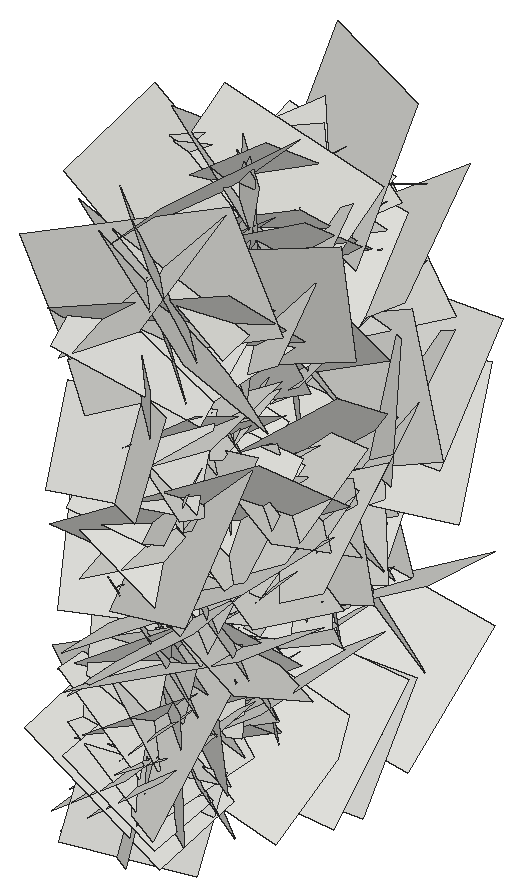
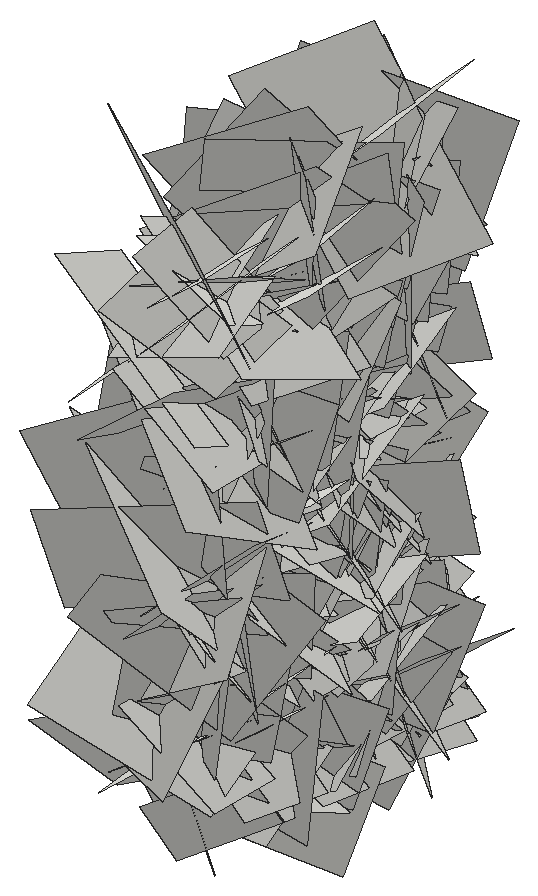
# SketchUp Ruby script. Lengths in inches.
U = 1.inch
M = Sketchup.active_model
def pt(a) = Geom::Point3d.new(a.map { |v| v * U })
def face(e, loops, mat)
  f = e.add_face(loops[0].map { |a| pt(a) })
  loops[1..].each { |l| e.add_face(l.map { |a| pt(a) }).erase! }
  f.material = f.back_material = mat if mat
  f
end
# faces: each face lists its corners as indices into pts; further lists are holes
def faces(e, pts, list, mat = nil) = list.each { |f| face(e, (f[0].is_a?(Array) ? f : [f]).map { |l| l.map { |i| pts[i] } }, mat) }
# xy, xz, yz: faces in a plane at the given z, y or x. An outline is a flat list of corners, or four numbers for a rectangle; further outlines are holes
def ring(l) = l.size == 4 ? [[l[0], l[1]], [l[2], l[1]], [l[2], l[3]], [l[0], l[3]]] : l.each_slice(2).to_a
def flat(e, list, mat, &to3) = list.each { |f| face(e, (f[0].is_a?(Array) ? f : [f]).map { |l| ring(l).map { |u, v| to3.(u, v) } }, mat) }
def xy(e, z, list, mat = nil) = flat(e, list, mat) { |x, y| [x, y, z] }
def xz(e, y, list, mat = nil) = flat(e, list, mat) { |x, z| [x, y, z] }
def yz(e, x, list, mat = nil) = flat(e, list, mat) { |y, z| [x, y, z] }
def lines(e, pts, list) = list.each { |a, b| e.add_line(pt(pts[a]), pt(pts[b])) }
# prism: a flat outline (further loops are holes) pulled along v
def prism(e, loops, v, mat = nil)
  f = face(e, loops, mat); d = Geom::Vector3d.new(v.map { |x| x * U })
  f.pushpull(f.normal.samedirection?(d) ? d.length : -d.length)
end
def box(e, o, s, mat = nil) = prism(e, [[o, [o[0] + s[0], o[1], o[2]], [o[0] + s[0], o[1] + s[1], o[2]], [o[0], o[1] + s[1], o[2]]]], [0, 0, s[2]], mat)
def at(x, y, z, deg = 0) = Geom::Transformation.translation(pt([x, y, z])) * Geom::Transformation.rotation(ORIGIN, Z_AXIS, deg.degrees)
def axes(o, x, y, z) = Geom::Transformation.new([*x, 0, *y, 0, *z, 0, *pt(o).to_a, 1])
def part(name) = M.definitions.add(name)
# library, detail: a bought-in or finely detailed component or shape, given as its bounding box
def library(name, o, s) = part(name).tap { |d| box(d.entities, o, s) }
def detail(e, o, s) = box(e.add_group.entities, o, s)
def put(e, d, t, mat = nil) = e.add_instance(d, t).tap { |i| i.material = mat if mat }
def group(e, t, mat = nil) = e.add_group.tap { |g| g.transformation = t; g.material = mat if mat }.entities
root = M.entities
c1 = part("Component\#6")
p = [[0.01,0,0],[0,3.24,4.54],[4.32,3.24,4.54],[4.33,0,0]]
faces(c1.entities,p,[[0,1,2,3]])
put(root,c1,axes([420.52,187.98,11.49],[-0.12716,0.81746,0.20835],[-0.15,0.18797,-0.81896],[0.88154,0.1499,-0.10929]))
put(root,c1,axes([420.52,186.0625,6.1],[-0.08854,0.52684,0.45627],[0.00383,0.45985,-0.53032],[0.73876,0.06076,0.05744]))
put(root,c1,axes([424.49,181.29,16.68],[-0.08133,-0.245,0.96212],[0.05676,0.96256,0.24939],[-1.05086,0.07095,-0.06099]))
put(root,c1,axes([424.49,184.19,13.53],[-0.08078,-0.49886,0.79857],[-0.01528,0.8017,0.49945],[-0.99796,0.02811,-0.07229]))
put(root,c1,axes([424.49,187.61,11.62],[0.28203,-0.58282,-1.12773],[-0.01249,-1.15332,0.59327],[-1.34554,-0.11146,-0.24188]))
put(root,c1,axes([420.52,183.1,18.89],[-0.1435,0.17311,-0.85276],[-0.14536,-0.85648,-0.1521],[0.91084,-0.10941,-0.15862]))
put(root,c1,axes([420.52,183.83,7.3125],[-0.02805,0.62389,-0.09529],[0.05665,-0.09282,-0.62253],[0.66659,0.03414,0.0489]))
put(root,c1,axes([424.49,184.51,1.15],[0.01173,-1.06899,-0.22188],[0.10644,-0.21996,1.06472],[-1.15237,-0.0312,0.09608]))
put(root,c1,axes([424.49,186.9375,3.03],[-0.11563,0.62873,-0.58509],[-0.05581,-0.59358,-0.62803],[-0.90867,-0.04354,0.11303]))
put(root,c1,axes([420.52,189.45,1.42],[0.1039,0.30381,0.53974],[-0.07033,0.54846,-0.29667],[0.65275,0.01074,-0.11787]))
put(root,c1,axes([420.52,184.54,3.47],[-0.05739,0.5962,-0.42459],[-0.0201,-0.42675,-0.59681],[0.77559,0.03305,-0.04688]))
put(root,c1,axes([424.49,185.64,19.96],[0.2349,1.07139,0.39402],[-0.08081,0.41437,-1.08385],[-1.20734,0.18072,0.1492]))
put(root,c1,axes([424.49,186.72,4.72],[0.08241,-0.91883,0.29273],[-0.13826,0.28096,0.91654],[-1.0128,-0.11312,-0.1013]))
put(root,c1,axes([424.49,190.33,17.67],[-0.17424,0.82504,0.17436],[0.04616,0.18571,-0.83769],[-0.89267,-0.15144,-0.07735]))
put(root,c1,axes([420.52,182.67,1.51],[-0.02969,-0.72745,-0.10184],[-0.03667,-0.1005,0.72735],[0.77775,-0.03251,0.03041]))
put(root,c1,axes([424.49,179.97,24.47],[0.23304,1.36821,0.06434],[0.25904,0.02493,-1.36533],[-1.42861,0.2277,-0.23708]))
put(root,c1,axes([420.52,184.43,15.42],[-0.12844,-0.04329,0.74472],[0.08874,0.74892,0.05716],[0.78574,-0.09166,0.11528]))
put(root,c1,axes([424.49,189.57,16.9],[-0.06471,0.53395,-0.71324],[-0.01751,-0.71546,-0.53421],[-0.94426,-0.02333,0.05878]))
put(root,c1,axes([424.49,191,16.96],[0.17643,-1.14926,-0.11809],[0.05518,-0.11173,1.16072],[-1.22339,-0.17078,0.03532]))
put(root,c1,axes([420.52,186.92,8.78],[-0.10246,-0.30095,0.75916],[-0.04625,0.76527,0.29782],[0.86439,0.00528,0.10592]))
put(root,c1,axes([424.49,180.14,11.99],[0.0212,0.75168,0.8023],[0.17372,0.79143,-0.74558],[-1.15236,0.13314,-0.09764]))
put(root,c1,axes([424.49,185.08,2.16],[-0.06404,-1.02262,-0.11109],[0.17979,-0.11966,1.00929],[-1.07543,0.04089,0.17535]))
put(root,c1,axes([424.49,187.17,12.95],[0.05814,-0.16279,1.09674],[0.14666,1.09051,0.15494],[-1.1661,0.12904,0.07417]))
put(root,c1,axes([424.49,187.85,22.99],[-0.09057,-0.06637,-0.91857],[0.07612,-0.92019,0.05981],[-0.97325,-0.06579,0.09016]))
put(root,c1,axes([420.52,183.375,2.21],[0.01982,-0.33114,-0.74136],[-0.16849,-0.7287,0.32148],[0.84401,-0.13769,0.08159]))
put(root,c1,axes([420.52,192.83,7.86],[0.1126,-0.65912,-0.17655],[-0.1088,-0.19208,0.65534],[0.71507,0.07456,0.12751]))
put(root,c1,axes([424.49,183.46,7.83],[0.1867,0.36795,-0.96583],[-0.13041,-0.96532,-0.39019],[-1.08777,0.17888,-0.11899]))
put(root,c1,axes([424.49,186.63,-0.64],[0.14781,-0.37723,1.01914],[0.01271,1.02797,0.37886],[-1.15185,-0.03706,0.13496]))
put(root,c1,axes([424.49,183.61,1.59],[-0.06331,-0.78644,0.46242],[0.03597,0.46118,0.7887],[-0.96639,0.06869,-0.00094]))
put(root,c1,axes([424.49,185.25,15.47],[-0.04372,0.77316,0.71524],[0.20224,0.70943,-0.75587],[-1.09798,0.09988,-0.16771]))
put(root,c1,axes([424.49,185.13,2.21],[-0.09174,0.69928,0.36],[-0.10121,0.35015,-0.7031],[-0.82753,-0.12035,0.04608]))
put(root,c1,axes([420.52,192.38,19.24],[0.04943,-0.7355,0.057],[-0.07325,0.05251,0.73407],[0.77853,0.05163,0.06545]))
put(root,c1,axes([424.49,181.6,11.88],[-0.05183,0.72565,0.67247],[0.15864,0.67097,-0.71314],[-1.03662,0.0664,-0.14276]))
put(root,c1,axes([420.52,185.26,12.26],[-0.159,0.84642,0.10737],[0.04855,0.11685,-0.85715],[0.9031,0.14274,0.06498]))
put(root,c1,axes([420.52,185.94,13.1875],[-0.12339,0.16979,-0.82402],[0.01755,-0.83125,-0.17361],[0.89164,0.03986,-0.11061]))
put(root,c1,axes([420.52,183.19,13.8],[-0.02762,0.65605,0.3231],[0.06014,0.32414,-0.6536],[0.77284,-0.00178,0.06241]))
put(root,c1,axes([424.49,184.53,11.29],[0.10396,-0.95246,0.37472],[0.04499,0.37989,0.95451],[-1.084,-0.07558,0.07555]))
put(root,c1,axes([424.49,192.08,20.31],[-0.05296,-0.67773,-0.30339],[-0.1724,-0.2867,0.66724],[-0.76797,0.11109,-0.12886]))
put(root,c1,axes([420.52,192.03,8.33],[-0.03388,0.22508,-0.86549],[-0.13142,-0.8588,-0.21876],[0.93879,-0.1121,-0.06186]))
put(root,c1,axes([420.52,185.14,8.49],[0.08576,-0.66072,-0.04627],[0.0456,-0.04128,0.66459],[0.70059,0.08356,-0.03759]))
put(root,c1,axes([420.52,183.28,17.73],[-0.09647,-0.26045,0.74001],[0.11879,0.73302,0.27177],[0.82305,-0.13632,0.04751]))
put(root,c1,axes([420.52,193.37,9.31],[-0.05697,-0.46717,-0.61186],[0.09106,-0.61316,0.46062],[0.81091,0.03603,-0.09471]))
put(root,c1,axes([420.52,191.46,9.82],[-0.08538,-0.06629,-0.92063],[-0.09555,-0.91915,0.07407],[0.97372,-0.09601,-0.07345]))
put(root,c1,axes([420.52,191.35,2.27],[-0.06694,-0.86655,-0.10749],[-0.04783,-0.10439,0.86806],[0.92435,-0.06816,0.03713]))
put(root,c1,axes([420.52,190.84,12.42],[0.00848,-0.77925,-0.15089],[-0.03038,-0.15108,0.77873],[0.8408,0.0024,0.02966]))
put(root,c1,axes([420.52,182.98,9.92],[0.09782,-0.62966,-0.10425],[0.08997,-0.09229,0.63256],[0.67052,0.10424,-0.06967]))
put(root,c1,axes([420.52,180.19,4.07],[0.08532,0.68038,-0.07405],[0.04058,-0.07892,-0.68351],[0.72433,-0.07573,0.04702]))
put(root,c1,axes([420.52,183.91,5.17],[-0.1157,0.58195,-0.7538],[-0.08085,-0.76164,-0.57696],[1.0062,0.00571,-0.13304]))
put(root,c1,axes([420.52,182.875,15.8],[-0.04284,-0.30855,-0.78276],[-0.017,-0.78324,0.30957],[0.8917,-0.02976,-0.0317]))
put(root,c1,axes([424.49,184.33,2.33],[0.23495,-0.78095,0.69461],[-0.033,0.70481,0.80235],[-1.10738,-0.18669,0.12346]))
put(root,c1,axes([424.49,189.86,21.06],[0.09411,0.75469,-0.30292],[-0.23058,-0.27158,-0.74036],[-0.83059,0.16091,0.17121]))
put(root,c1,axes([424.49,189.65,5.54],[-0.06955,0.77959,0.08211],[-0.00823,0.08175,-0.78235],[-0.8309,-0.06607,0.00087]))
put(root,c1,axes([424.49,192.04,5.47],[0.24252,-0.79203,0.72828],[0.0092,0.7459,0.80846],[-1.14049,-0.1624,0.16139]))
put(root,c1,axes([424.49,184.16,21.8125],[0.07155,0.99261,-0.10082],[0.11355,-0.10768,-0.9884],[-1.05147,0.05592,-0.1136]))
put(root,c1,axes([420.52,184.68,7.1],[-0.07537,-0.21143,-0.85755],[-0.01444,-0.85996,0.21315],[0.93612,-0.03029,-0.06575]))
put(root,c1,axes([420.52,187.95,18.35],[-0.24952,-0.85217,0.60628],[-0.01294,0.62364,0.87183],[1.1085,-0.18454,0.14665]))
put(root,c1,axes([424.49,188.38,23.95],[0.14683,-0.05211,-1.06804],[0.1506,-1.06652,0.07046],[-1.12342,-0.14978,-0.13015]))
put(root,c1,axes([420.52,188.38,23.95],[-0.14683,-0.05211,-1.06804],[-0.1506,-1.06652,0.07046],[1.12342,-0.14978,-0.13015]))
put(root,c1,axes([424.49,187.95,18.35],[0.24952,-0.85217,0.60628],[0.01294,0.62364,0.87183],[-1.1085,-0.18454,0.14665]))
put(root,c1,axes([424.49,184.68,7.1],[0.07537,-0.21143,-0.85755],[0.01444,-0.85996,0.21315],[-0.93612,-0.03029,-0.06575]))
put(root,c1,axes([420.52,184.16,21.8125],[-0.07155,0.99261,-0.10082],[-0.11355,-0.10768,-0.9884],[1.05147,0.05592,-0.1136]))
put(root,c1,axes([420.52,192.04,5.47],[-0.24252,-0.79203,0.72828],[-0.0092,0.7459,0.80846],[1.14049,-0.1624,0.16139]))
put(root,c1,axes([420.52,189.65,5.54],[0.06955,0.77959,0.08211],[0.00823,0.08175,-0.78235],[0.8309,-0.06607,0.00087]))
put(root,c1,axes([420.52,189.86,21.06],[-0.09411,0.75469,-0.30292],[0.23058,-0.27158,-0.74036],[0.83059,0.16091,0.17121]))
put(root,c1,axes([420.52,184.33,2.33],[-0.23495,-0.78095,0.69461],[0.033,0.70481,0.80235],[1.10738,-0.18669,0.12346]))
put(root,c1,axes([424.49,182.875,15.8],[0.04284,-0.30855,-0.78276],[0.017,-0.78324,0.30957],[-0.8917,-0.02976,-0.0317]))
put(root,c1,axes([424.49,183.91,5.17],[0.1157,0.58195,-0.7538],[0.08085,-0.76164,-0.57696],[-1.0062,0.00571,-0.13304]))
put(root,c1,axes([424.49,180.19,4.07],[-0.08532,0.68038,-0.07405],[-0.04058,-0.07892,-0.68351],[-0.72433,-0.07573,0.04702]))
put(root,c1,axes([424.49,182.98,9.92],[-0.09782,-0.62966,-0.10425],[-0.08997,-0.09229,0.63256],[-0.67052,0.10424,-0.06967]))
put(root,c1,axes([424.49,190.84,12.42],[-0.00848,-0.77925,-0.15089],[0.03038,-0.15108,0.77873],[-0.8408,0.0024,0.02966]))
put(root,c1,axes([424.49,191.35,2.27],[0.06694,-0.86655,-0.10749],[0.04783,-0.10439,0.86806],[-0.92435,-0.06816,0.03713]))
put(root,c1,axes([424.49,191.46,9.82],[0.08538,-0.06629,-0.92063],[0.09555,-0.91915,0.07407],[-0.97372,-0.09601,-0.07345]))
put(root,c1,axes([424.49,193.37,9.31],[0.05697,-0.46717,-0.61186],[-0.09106,-0.61316,0.46062],[-0.81091,0.03603,-0.09471]))
put(root,c1,axes([424.49,183.28,17.73],[0.09647,-0.26045,0.74001],[-0.11879,0.73302,0.27177],[-0.82305,-0.13632,0.04751]))
put(root,c1,axes([424.49,185.14,8.49],[-0.08576,-0.66072,-0.04627],[-0.0456,-0.04128,0.66459],[-0.70059,0.08356,-0.03759]))
put(root,c1,axes([424.49,192.03,8.33],[0.03388,0.22508,-0.86549],[0.13142,-0.8588,-0.21876],[-0.93879,-0.1121,-0.06186]))
put(root,c1,axes([420.52,192.08,20.31],[0.05296,-0.67773,-0.30339],[0.1724,-0.2867,0.66724],[0.76797,0.11109,-0.12886]))
put(root,c1,axes([420.52,184.53,11.29],[-0.10396,-0.95246,0.37472],[-0.04499,0.37989,0.95451],[1.084,-0.07558,0.07555]))
put(root,c1,axes([424.49,183.19,13.8],[0.02762,0.65605,0.3231],[-0.06014,0.32414,-0.6536],[-0.77284,-0.00178,0.06241]))
put(root,c1,axes([424.49,185.94,13.1875],[0.12339,0.16979,-0.82402],[-0.01755,-0.83125,-0.17361],[-0.89164,0.03986,-0.11061]))
put(root,c1,axes([424.49,185.26,12.26],[0.159,0.84642,0.10737],[-0.04855,0.11685,-0.85715],[-0.9031,0.14274,0.06498]))
put(root,c1,axes([420.52,181.6,11.88],[0.05183,0.72565,0.67247],[-0.15864,0.67097,-0.71314],[1.03662,0.0664,-0.14276]))
put(root,c1,axes([424.49,192.38,19.24],[-0.04943,-0.7355,0.057],[0.07325,0.05251,0.73407],[-0.77853,0.05163,0.06545]))
put(root,c1,axes([420.52,185.13,2.21],[0.09174,0.69928,0.36],[0.10121,0.35015,-0.7031],[0.82753,-0.12035,0.04608]))
put(root,c1,axes([420.52,185.25,15.47],[0.04372,0.77316,0.71524],[-0.20224,0.70943,-0.75587],[1.09798,0.09988,-0.16771]))
put(root,c1,axes([420.52,183.61,1.59],[0.06331,-0.78644,0.46242],[-0.03597,0.46118,0.7887],[0.96639,0.06869,-0.00094]))
put(root,c1,axes([420.52,186.63,-0.64],[-0.14781,-0.37723,1.01914],[-0.01271,1.02797,0.37886],[1.15185,-0.03706,0.13496]))
put(root,c1,axes([420.52,183.46,7.83],[-0.1867,0.36795,-0.96583],[0.13041,-0.96532,-0.39019],[1.08777,0.17888,-0.11899]))
put(root,c1,axes([424.49,192.83,7.86],[-0.1126,-0.65912,-0.17655],[0.1088,-0.19208,0.65534],[-0.71507,0.07456,0.12751]))
put(root,c1,axes([424.49,183.375,2.21],[-0.01982,-0.33114,-0.74136],[0.16849,-0.7287,0.32148],[-0.84401,-0.13769,0.08159]))
put(root,c1,axes([420.52,187.85,22.99],[0.09057,-0.06637,-0.91857],[-0.07612,-0.92019,0.05981],[0.97325,-0.06579,0.09016]))
put(root,c1,axes([420.52,187.17,12.95],[-0.05814,-0.16279,1.09674],[-0.14666,1.09051,0.15494],[1.1661,0.12904,0.07417]))
put(root,c1,axes([420.52,185.08,2.16],[0.06404,-1.02262,-0.11109],[-0.17979,-0.11966,1.00929],[1.07543,0.04089,0.17535]))
put(root,c1,axes([420.52,180.14,11.99],[-0.0212,0.75168,0.8023],[-0.17372,0.79143,-0.74558],[1.15236,0.13314,-0.09764]))
put(root,c1,axes([424.49,186.92,8.78],[0.10246,-0.30095,0.75916],[0.04625,0.76527,0.29782],[-0.86439,0.00528,0.10592]))
put(root,c1,axes([420.52,191,16.96],[-0.17643,-1.14926,-0.11809],[-0.05518,-0.11173,1.16072],[1.22339,-0.17078,0.03532]))
put(root,c1,axes([420.52,189.57,16.9],[0.06471,0.53395,-0.71324],[0.01751,-0.71546,-0.53421],[0.94426,-0.02333,0.05878]))
put(root,c1,axes([424.49,184.43,15.42],[0.12844,-0.04329,0.74472],[-0.08874,0.74892,0.05716],[-0.78574,-0.09166,0.11528]))
put(root,c1,axes([420.52,179.97,24.47],[-0.23304,1.36821,0.06434],[-0.25904,0.02493,-1.36533],[1.42861,0.2277,-0.23708]))
put(root,c1,axes([424.49,182.67,1.51],[0.02969,-0.72745,-0.10184],[0.03667,-0.1005,0.72735],[-0.77775,-0.03251,0.03041]))
put(root,c1,axes([420.52,190.33,17.67],[0.17424,0.82504,0.17436],[-0.04616,0.18571,-0.83769],[0.89267,-0.15144,-0.07735]))
put(root,c1,axes([420.52,186.72,4.72],[-0.08241,-0.91883,0.29273],[0.13826,0.28096,0.91654],[1.0128,-0.11312,-0.1013]))
put(root,c1,axes([420.52,185.64,19.96],[-0.2349,1.07139,0.39402],[0.08081,0.41437,-1.08385],[1.20734,0.18072,0.1492]))
put(root,c1,axes([424.49,184.54,3.47],[0.05739,0.5962,-0.42459],[0.0201,-0.42675,-0.59681],[-0.77559,0.03305,-0.04688]))
put(root,c1,axes([424.49,189.45,1.42],[-0.1039,0.30381,0.53974],[0.07033,0.54846,-0.29667],[-0.65275,0.01074,-0.11787]))
put(root,c1,axes([420.52,186.9375,3.03],[0.11563,0.62873,-0.58509],[0.05581,-0.59358,-0.62803],[0.90867,-0.04354,0.11303]))
put(root,c1,axes([420.52,184.51,1.15],[-0.01173,-1.06899,-0.22188],[-0.10644,-0.21996,1.06472],[1.15237,-0.0312,0.09608]))
put(root,c1,axes([424.49,183.83,7.3125],[0.02805,0.62389,-0.09529],[-0.05665,-0.09282,-0.62253],[-0.66659,0.03414,0.0489]))
put(root,c1,axes([424.49,183.1,18.89],[0.1435,0.17311,-0.85276],[0.14536,-0.85648,-0.1521],[-0.91084,-0.10941,-0.15862]))
put(root,c1,axes([420.52,187.61,11.62],[-0.28203,-0.58282,-1.12773],[0.01249,-1.15332,0.59327],[1.34554,-0.11146,-0.24188]))
put(root,c1,axes([420.52,184.19,13.53],[0.08078,-0.49886,0.79857],[0.01528,0.8017,0.49945],[0.99796,0.02811,-0.07229]))
put(root,c1,axes([420.52,181.29,16.68],[0.08133,-0.245,0.96212],[-0.05676,0.96256,0.24939],[1.05086,0.07095,-0.06099]))
put(root,c1,axes([424.49,186.0625,6.1],[0.08854,0.52684,0.45627],[-0.00383,0.45985,-0.53032],[-0.73876,0.06076,0.05744]))
put(root,c1,axes([424.49,187.98,11.49],[0.12716,0.81746,0.20835],[0.15,0.18797,-0.81896],[-0.88154,0.1499,-0.10929]))
put(root,c1,axes([420.52,194.3,13.93],[-0.22437,-1.23478,-0.60854],[-0.19245,-0.58527,1.25072],[1.44644,-0.26941,0.07201]))
put(root,c1,axes([420.52,184.41,20.14],[-0.03821,-1.03167,-0.60174],[-0.15497,-0.59368,1.0266],[1.25647,-0.1046,0.10832]))
put(root,c1,axes([424.49,186.3,8.38],[-0.07617,0.47932,0.41871],[0.13681,0.42359,-0.46276],[-0.66062,0.03245,-0.14411]))
put(root,c1,axes([420.52,184.31,4.6],[0.1576,-0.1516,-1.0147],[-0.15202,-1.0183,0.13112],[1.07684,-0.12157,0.16702]))
put(root,c1,axes([420.52,179.32,18.3],[0.15069,0.54422,0.74866],[-0.00735,0.75804,-0.54972],[0.98107,-0.07791,-0.11911]))
put(root,c1,axes([424.49,188.8,6.44],[0.14743,-0.18272,-0.74199],[0.06403,-0.74919,0.19581],[-0.80747,-0.09277,-0.11994]))
put(root,c1,axes([420.52,185.52,6.2],[-0.2751,-0.65276,-1.16933],[-0.03559,-1.18754,0.67037],[1.41909,-0.15632,-0.20987]))
put(root,c1,axes([420.52,181.08,20.02],[-0.00536,1.00575,0.03656],[0.10796,0.03689,-1.00058],[1.06133,0.00133,0.10197]))
put(root,c1,axes([420.52,184.05,20.67],[0.10102,0.73684,0.6989],[-0.04073,0.70408,-0.73707],[1.07574,-0.04254,-0.09354]))
put(root,c1,axes([420.52,191.125,9.45],[-0.23474,-0.88576,-0.93612],[0.00151,-0.95001,0.89856],[1.36608,-0.15116,-0.16185]))
put(root,c1,axes([420.52,185.11,13.22],[0.08906,-0.95701,-0.12674],[0.0585,-0.12225,0.95969],[1.02162,0.09043,-0.0439]))
put(root,c1,axes([420.52,180.4,17.125],[-0.23878,-0.31981,1.17522],[0.15258,1.17979,0.34864],[1.28199,-0.19998,0.17739]))
put(root,c1,axes([420.52,187.48,17.59],[-0.04794,-0.78864,0.66349],[0.19289,0.64758,0.78214],[1.07529,-0.15133,-0.11072]))
put(root,c1,axes([420.52,187.26,9.21],[0.06299,-0.71122,-0.64775],[0.16214,-0.63375,0.70987],[1.00673,0.14657,-0.0738]))
put(root,c1,axes([424.49,191.11,1.26],[0.04561,-0.57908,-0.31344],[0.1156,-0.3035,0.57569],[-0.68833,-0.08935,0.07592]))
put(root,c1,axes([420.52,186.13,19.34],[0.13168,0.96657,0.23982],[0.01085,0.24043,-0.97432],[1.05558,-0.12304,-0.0199]))
put(root,c1,axes([420.52,185.36,5.79],[0.02078,-1.22604,-0.15411],[-0.11589,-0.15525,1.22117],[1.3047,0.00574,0.11093]))
put(root,c1,axes([420.52,186.43,6.6],[-0.00451,1.27416,-0.10814],[-0.14001,-0.108,-1.26731],[1.34821,-0.00695,-0.13197]))
put(root,c1,axes([424.49,190.35,18.26],[0.16101,-0.65287,0.16772],[0.08445,0.18811,0.66008],[-0.7095,-0.12576,0.11663]))
put(root,c1,axes([420.52,187.9375,5.11],[0.04973,-1.23753,-0.07043],[-0.13139,-0.07481,1.23194],[1.30732,0.03956,0.12649]))
put(root,c1,axes([420.52,189.08,9.2],[-0.13088,0.55221,1.09741],[0.12619,1.10312,-0.54169],[1.29609,-0.05164,0.16356]))
put(root,c1,axes([420.52,182.44,13.63],[-0.1579,1.28482,-0.45217],[-0.02165,-0.45692,-1.2916],[1.44363,0.13368,-0.06883]))
put(root,c1,axes([420.52,182.53,23.48],[0.24403,0.37129,-0.99391],[-0.1038,-1.00526,-0.39821],[1.11985,-0.17408,0.17968]))
put(root,c1,axes([420.52,192.17,8.01],[0.17438,0.53527,-0.89237],[0.02164,-0.90494,-0.53904],[1.10282,-0.06688,0.15168]))
put(root,c1,axes([420.52,188.23,7.57],[0.0913,-1.12353,0.75234],[-0.27462,0.72618,1.11413],[1.40673,0.21468,0.16867]))
put(root,c1,axes([420.52,194.04,23.84],[-0.15699,-0.54259,-1.24113],[0.03696,-1.24964,0.54215],[1.43535,-0.02717,-0.14971]))
put(root,c1,axes([420.52,189.36,1.43],[-0.09807,-1.35815,-0.14277],[-0.05055,-0.1398,1.36078],[1.44669,-0.09695,0.03787]))
put(root,c1,axes([420.52,188.7,21.97],[0.14471,1.28216,-0.28655],[-0.25359,-0.25902,-1.27293],[1.36933,-0.18346,-0.20546]))
put(root,c1,axes([420.52,190.12,11.53],[-0.21117,-0.99907,-0.90649],[0.1512,-0.92678,0.99009],[1.42194,-0.04983,-0.2399]))
put(root,c1,axes([420.52,183.02,16.38],[-0.02893,-0.8566,0.75588],[0.26219,0.73373,0.84043],[1.18223,-0.18368,-0.16789]))
put(root,c1,axes([420.52,185.31,6.45],[-0.03902,-0.20515,1.15818],[0.22164,1.13915,0.20842],[1.22693,-0.21231,-0.00082]))
put(root,c1,axes([420.52,180.93,10.86],[-0.17521,1.15715,-0.62152],[0.20897,-0.59747,-1.1648],[1.37654,0.23798,0.09772]))
put(root,c1,axes([420.52,184.5,10.44],[0.20009,0.552,-0.98447],[-0.02572,-0.99592,-0.56307],[1.1961,-0.11375,0.15258]))
put(root,c1,axes([420.52,185.25,0.97],[0.15144,0.45294,1.0525],[0.02813,1.05906,-0.45936],[1.21425,-0.08102,-0.12063]))
put(root,c1,axes([420.52,182.38,2.76],[0.16715,0.82367,0.72398],[0.09449,0.71938,-0.83785],[1.15857,-0.1775,-0.03612]))
put(root,c1,axes([420.52,186.66,10.07],[-0.09303,-0.2424,1.37134],[-0.00293,1.37409,0.24271],[1.47615,-0.01254,0.08691]))
put(root,c1,axes([420.52,192.77,15.58],[0.03721,-0.16955,-1.17702],[0.1418,-1.1695,0.17246],[1.25252,0.13744,0.01545]))
put(root,c1,axes([420.52,185.87,11.99],[0.00632,-0.88407,-1.06115],[-0.10628,-1.05864,0.88141],[1.46017,-0.07323,0.06874]))
put(root,c1,axes([420.52,186.02,17.55],[0.12484,-0.91824,0.67786],[0.09261,0.68671,0.91505],[1.20627,0.04231,-0.14041]))
put(root,c1,axes([420.52,195.54,11.625],[0.04246,-1.00606,-0.92627],[-0.11693,-0.92602,1.00103],[1.44486,-0.04538,0.10823]))
put(root,c1,axes([420.52,183.88,15.08],[-0.0404,1.11797,-0.62329],[0.16276,-0.61507,-1.11262],[1.34698,0.10785,0.11575]))
put(root,c1,axes([420.52,184.23,21.55],[0.30098,0.54789,0.85036],[0.10123,0.86476,-0.58905],[1.06749,-0.23649,-0.1839]))
put(root,c1,axes([420.52,184,8.18],[-0.02134,-1.06466,0.81449],[0.04088,0.81378,1.06469],[1.42032,-0.03942,-0.01841]))
put(root,c1,axes([420.52,188.34,12.62],[0.20954,0.481,1.15591],[-0.07101,1.17261,-0.47649],[1.32521,-0.01322,-0.2083]))
put(root,c1,axes([420.52,186.39,13.5625],[0.22643,-0.80881,0.81079],[0.0736,0.83241,0.81208],[1.21171,0.10058,-0.20084]))
put(root,c1,axes([420.52,184.34,4.6],[0.11485,-1.15497,0.26483],[0.19184,0.27894,1.14248],[1.2413,0.06375,-0.20107]))
put(root,c1,axes([420.52,193.03,3.2],[0.23388,-1.096,0.27231],[0.13541,0.2999,1.10354],[1.1894,0.18138,-0.17918]))
put(root,c1,axes([420.52,189.55,17.94],[0.16397,-1.09761,-0.83604],[-0.11999,-0.84854,1.09307],[1.45761,0.05363,0.18403]))
put(root,c1,axes([420.52,187.39,3.1875],[0.10139,0.89849,0.89189],[0.1671,0.87902,-0.90243],[1.33152,-0.17873,0.04534]))
put(root,c1,axes([420.52,180.76,23.09],[0.06995,0.91309,-0.96842],[0.10566,-0.97028,-0.90805],[1.4069,0.02747,0.11634]))
put(root,c1,axes([420.52,183.54,2.14],[0.03864,0.84179,0.92004],[0.33491,0.88417,-0.82148],[1.27872,-0.257,0.18735]))
put(root,c1,axes([420.52,184.58,6.82],[0.16596,-1.29847,0.14138],[0.0614,0.14916,1.30572],[1.38315,0.14917,-0.07492]))
put(root,c1,axes([420.52,193.85,16.74],[0.30124,-1.14539,-0.57535],[-0.00001,-0.58933,1.17321],[1.35869,0.25394,0.12757]))
put(root,c1,axes([420.52,189.11,8.53],[0.25892,-1.11224,-0.53402],[0.14932,-0.51568,1.13849],[1.29927,0.28091,-0.02442]))
put(root,c1,axes([420.52,182.27,16.13],[0.23771,-0.47409,1.27281],[0.00404,1.29026,0.47991],[1.43973,0.07465,-0.2115]))
